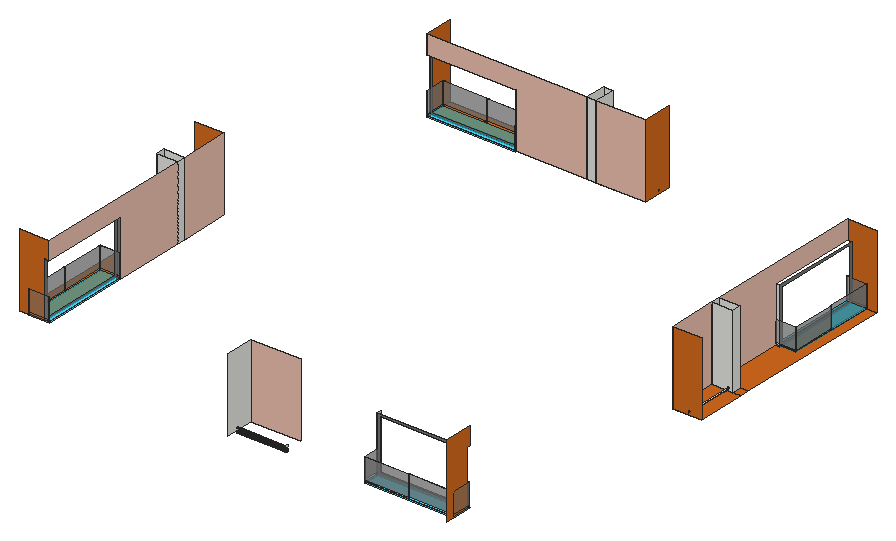
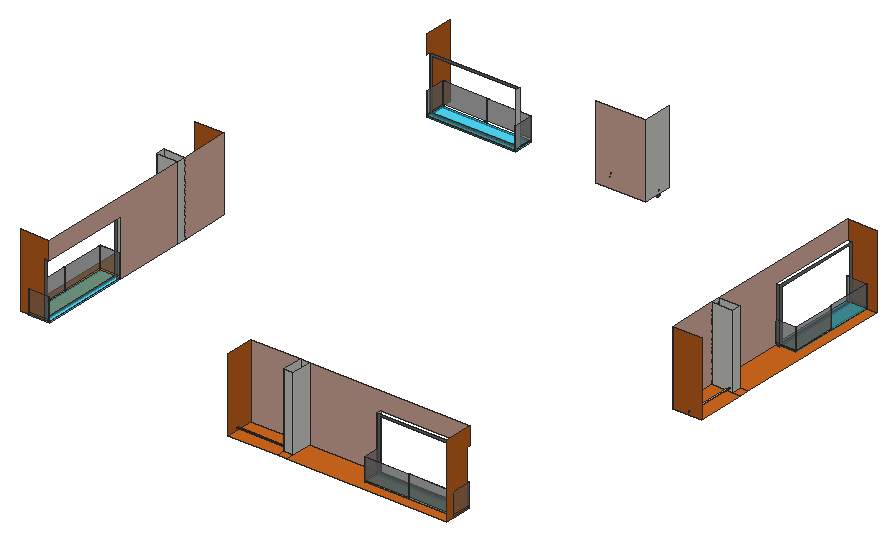
# SketchUp Ruby script. Lengths in inches.
U = 1.inch
M = Sketchup.active_model
def pt(a) = Geom::Point3d.new(a.map { |v| v * U })
def face(e, loops, mat)
  f = e.add_face(loops[0].map { |a| pt(a) })
  loops[1..].each { |l| e.add_face(l.map { |a| pt(a) }).erase! }
  f.material = f.back_material = mat if mat
  f
end
# faces: each face lists its corners as indices into pts; further lists are holes
def faces(e, pts, list, mat = nil) = list.each { |f| face(e, (f[0].is_a?(Array) ? f : [f]).map { |l| l.map { |i| pts[i] } }, mat) }
# xy, xz, yz: faces in a plane at the given z, y or x. An outline is a flat list of corners, or four numbers for a rectangle; further outlines are holes
def ring(l) = l.size == 4 ? [[l[0], l[1]], [l[2], l[1]], [l[2], l[3]], [l[0], l[3]]] : l.each_slice(2).to_a
def flat(e, list, mat, &to3) = list.each { |f| face(e, (f[0].is_a?(Array) ? f : [f]).map { |l| ring(l).map { |u, v| to3.(u, v) } }, mat) }
def xy(e, z, list, mat = nil) = flat(e, list, mat) { |x, y| [x, y, z] }
def xz(e, y, list, mat = nil) = flat(e, list, mat) { |x, z| [x, y, z] }
def yz(e, x, list, mat = nil) = flat(e, list, mat) { |y, z| [x, y, z] }
def lines(e, pts, list) = list.each { |a, b| e.add_line(pt(pts[a]), pt(pts[b])) }
# prism: a flat outline (further loops are holes) pulled along v
def prism(e, loops, v, mat = nil)
  f = face(e, loops, mat); d = Geom::Vector3d.new(v.map { |x| x * U })
  f.pushpull(f.normal.samedirection?(d) ? d.length : -d.length)
end
def box(e, o, s, mat = nil) = prism(e, [[o, [o[0] + s[0], o[1], o[2]], [o[0] + s[0], o[1] + s[1], o[2]], [o[0], o[1] + s[1], o[2]]]], [0, 0, s[2]], mat)
def at(x, y, z, deg = 0) = Geom::Transformation.translation(pt([x, y, z])) * Geom::Transformation.rotation(ORIGIN, Z_AXIS, deg.degrees)
def axes(o, x, y, z) = Geom::Transformation.new([*x, 0, *y, 0, *z, 0, *pt(o).to_a, 1])
def part(name) = M.definitions.add(name)
# library, detail: a bought-in or finely detailed component or shape, given as its bounding box
def library(name, o, s) = part(name).tap { |d| box(d.entities, o, s) }
def detail(e, o, s) = box(e.add_group.entities, o, s)
def put(e, d, t, mat = nil) = e.add_instance(d, t).tap { |i| i.material = mat if mat }
def group(e, t, mat = nil) = e.add_group.tap { |g| g.transformation = t; g.material = mat if mat }.entities
root = M.entities
M.materials.add("[0041_Chocolate]").color = [210, 105, 30]
M.materials.add("[0042_Sienna]").color = [160, 82, 45]
M.materials.add("[0119_RosyBrown]").color = [234, 190, 174]
M.materials.add("[Metal Seamed]").color = [118, 119, 115]
M.materials.add("[Translucent Glass Tinted]").color = [8, 201, 241]
M.materials["[Translucent Glass Tinted]"].alpha = 0.48
M.materials.add("[Translucent_Glass_Gray]").color = [128, 128, 128]
M.materials["[Translucent_Glass_Gray]"].alpha = 0.5
c1 = part("Altan")
box(c1.entities,[0,0,0],[118.11,59.06,3.9375])
c2 = part("Staal sojle alta")
box(c2.entities,[0,0,0],[0.87,0.87,43.31])
c3 = part("gler")
box(c3.entities,[0,-0.71,0],[0.37,57.8,41.34],"[Translucent_Glass_Gray]")
xy(root,1573.11,[[72,636.29,132,662.8],[1488,886.83,1548,913.33],[671.48,1452.8125,697.99,1512.8125]])
xy(root,1573.11,[[48,169.92,120,169.92,120,429.61,132,429.61,132,636.29,48,636.29],[48,636.29,72,662.8],[48,662.8,132,806.17],[1488,743.45,1572,886.83],[1548,886.83,1572,913.33],
  [1488,913.33,1572,913.33,1572,1379.7,1500,1379.7,1500,1120.01,1488,1120.01],[464.8,1452.8125,671.48,1452.8125,671.48,1536.8125,205.11,1536.8125,205.11,1464.8125,464.8,1464.8125],[697.99,1452.8125,841.36,1536.8125],[671.48,1512.8125,697.99,1536.8125]],"[0041_Chocolate]")
xy(root,1573.11,[[1155.2,84.8125,1414.89,96.8125]],"[0042_Sienna]")
xz(root,84.8125,[[[1155.2,1573.11,1414.89,1733.61],[1161.2,1579.11,1408.89,1727.61]]],"[Metal Seamed]")
xz(root,96.8125,[[778.64,1573.11,922.01,1786.89]],"[0119_RosyBrown]")
xz(root,169.92,[[48,1573.11,48,1786.89,132,1786.89,132,1733.61,120,1733.61,120,1573.11]],"[0041_Chocolate]")
xz(root,429.61,[[120,1573.11,132,1733.61]],"[Metal Seamed]")
xz(root,636.29,[[72,1573.11,132,1786.89]])
xz(root,662.8,[[[72,1573.11,132,1786.89],[83.53,1578.02,84.48,1578.14,85.37,1578.51,86.13,1579.1,86.72,1579.86,87.09,1580.75,87.21,1581.7,87.09,1582.66,86.72,1583.55,86.13,1584.3125,85.37,1584.9,84.48,1585.27,83.53,1585.39,82.57,1585.27,81.68,1584.9,80.92,1584.3125,80.33,1583.55,79.97,1582.66,79.84,1581.7,79.97,1580.75,80.33,1579.86,80.92,1579.1,81.68,1578.51,82.57,1578.14]],[83.53,1578.02,84.48,1578.14,85.37,1578.51,86.13,1579.1,86.72,1579.86,87.09,1580.75,87.21,1581.7,87.09,1582.66,86.72,1583.55,86.13,1584.3125,85.37,1584.9,84.48,1585.27,83.53,1585.39,82.57,1585.27,81.68,1584.9,80.92,1584.3125,80.33,1583.55,79.97,1582.66,79.84,1581.7,79.97,1580.75,80.33,1579.86,80.92,1579.1,81.68,1578.51,82.57,1578.14]])
xz(root,743.45,[[[1488,1573.11,1572,1786.89],[1536.47,1578.02,1537.43,1578.14,1538.32,1578.51,1539.08,1579.1,1539.67,1579.86,1540.03,1580.75,1540.16,1581.7,1540.03,1582.66,1539.67,1583.55,1539.08,1584.3125,1538.32,1584.9,1537.43,1585.27,1536.47,1585.39,1535.52,1585.27,1534.63,1584.9,1533.87,1584.3125,1533.28,1583.55,1532.91,1582.66,1532.79,1581.7,1532.91,1580.75,1533.28,1579.86,1533.87,1579.1,1534.63,1578.51,1535.52,1578.14]]],"[0041_Chocolate]")
xz(root,806.17,[[[48,1573.11,132,1786.89],[83.53,1578.02,82.57,1578.14,81.68,1578.51,80.92,1579.1,80.33,1579.86,79.97,1580.75,79.84,1581.7,79.97,1582.66,80.33,1583.55,80.92,1584.3125,81.68,1584.9,82.57,1585.27,83.53,1585.39,84.48,1585.27,85.37,1584.9,86.13,1584.3125,86.72,1583.55,87.09,1582.66,87.21,1581.7,87.09,1580.75,86.72,1579.86,86.13,1579.1,85.37,1578.51,84.48,1578.14]]],"[0041_Chocolate]")
xz(root,886.83,[[[1488,1573.11,1548,1786.89],[1536.47,1578.02,1535.52,1578.14,1534.63,1578.51,1533.87,1579.1,1533.28,1579.86,1532.91,1580.75,1532.79,1581.7,1532.91,1582.66,1533.28,1583.55,1533.87,1584.3125,1534.63,1584.9,1535.52,1585.27,1536.47,1585.39,1537.43,1585.27,1538.32,1584.9,1539.08,1584.3125,1539.67,1583.55,1540.03,1582.66,1540.16,1581.7,1540.03,1580.75,1539.67,1579.86,1539.08,1579.1,1538.32,1578.51,1537.43,1578.14]],[1536.47,1578.02,1535.52,1578.14,1534.63,1578.51,1533.87,1579.1,1533.28,1579.86,1532.91,1580.75,1532.79,1581.7,1532.91,1582.66,1533.28,1583.55,1533.87,1584.3125,1534.63,1584.9,1535.52,1585.27,1536.47,1585.39,1537.43,1585.27,1538.32,1584.9,1539.08,1584.3125,1539.67,1583.55,1540.03,1582.66,1540.16,1581.7,1540.03,1580.75,1539.67,1579.86,1539.08,1579.1,1538.32,1578.51,1537.43,1578.14]])
xz(root,913.33,[[1488,1573.11,1548,1786.89]])
xz(root,1120.01,[[1488,1573.11,1500,1733.61]])
xz(root,1379.7,[[1500,1573.11,1572,1573.11,1572,1786.89,1488,1786.89,1488,1733.61,1500,1733.61]],"[0041_Chocolate]")
xz(root,1452.8125,[[671.48,1573.11,697.99,1786.89]])
xz(root,1452.8125,[[464.8,1573.11,464.8,1733.61,205.11,1733.61,205.11,1786.89,671.48,1786.89,671.48,1573.11],[697.99,1573.11,841.36,1786.89]],"[0119_RosyBrown]")
xz(root,1464.8125,[[[205.11,1573.11,464.8,1733.61],[211.11,1579.11,458.8,1727.61]]],"[Metal Seamed]")
xz(root,1512.8125,[[671.48,1573.11,697.99,1786.89]])
yz(root,72,[[636.29,1573.11,662.8,1786.89]])
yz(root,120,[[[169.92,1573.11,429.61,1733.61],[175.92,1579.11,423.61,1727.61]]],"[Metal Seamed]")
yz(root,132,[[636.29,1573.11,662.8,1786.89]])
yz(root,132,[[429.61,1573.11,429.61,1733.61,169.92,1733.61,169.92,1786.89,636.29,1786.89,636.29,1573.11],[662.8,1573.11,806.17,1786.89]],"[0119_RosyBrown]")
yz(root,205.11,[[1464.8125,1573.11,1536.8125,1573.11,1536.8125,1786.89,1452.8125,1786.89,1452.8125,1733.61,1464.8125,1733.61]],"[0041_Chocolate]")
yz(root,464.8,[[1452.8125,1573.11,1464.8125,1733.61]])
yz(root,671.48,[[1452.8125,1573.11,1512.8125,1786.89]])
yz(root,697.99,[[[1452.8125,1573.11,1512.8125,1786.89],[1501.28,1578.02,1500.33,1578.14,1499.44,1578.51,1498.68,1579.1,1498.09,1579.86,1497.72,1580.75,1497.6,1581.7,1497.72,1582.66,1498.09,1583.55,1498.68,1584.3125,1499.44,1584.9,1500.33,1585.27,1501.28,1585.39,1502.24,1585.27,1503.13,1584.9,1503.89,1584.3125,1504.48,1583.55,1504.85,1582.66,1504.97,1581.7,1504.85,1580.75,1504.48,1579.86,1503.89,1579.1,1503.13,1578.51,1502.24,1578.14]],[1501.28,1578.02,1500.33,1578.14,1499.44,1578.51,1498.68,1579.1,1498.09,1579.86,1497.72,1580.75,1497.6,1581.7,1497.72,1582.66,1498.09,1583.55,1498.68,1584.3125,1499.44,1584.9,1500.33,1585.27,1501.28,1585.39,1502.24,1585.27,1503.13,1584.9,1503.89,1584.3125,1504.48,1583.55,1504.85,1582.66,1504.97,1581.7,1504.85,1580.75,1504.48,1579.86,1503.89,1579.1,1503.13,1578.51,1502.24,1578.14]])
yz(root,778.64,[[[12.8125,1573.11,47.01,1573.11,47.38,1573.27,48.34,1573.39,49.29,1573.27,49.67,1573.11,96.8125,1573.11,96.8125,1786.89,12.8125,1786.89],[48.34,1578.02,47.38,1578.14,46.5,1578.51,45.73,1579.1,45.15,1579.86,44.78,1580.75,44.65,1581.7,44.78,1582.66,45.15,1583.55,45.73,1584.3125,46.5,1584.9,47.38,1585.27,48.34,1585.39,49.29,1585.27,50.18,1584.9,50.95,1584.3125,51.53,1583.55,51.9,1582.66,52.03,1581.7,51.9,1580.75,51.53,1579.86,50.95,1579.1,50.18,1578.51,49.29,1578.14]],[47.01,1573.11,49.67,1573.11,49.29,1573.27,48.34,1573.39,47.38,1573.27]])
yz(root,778.64,[[48.34,1566.02,49.29,1566.14,50.18,1566.51,50.95,1567.1,51.53,1567.86,51.9,1568.75,52.03,1569.7,51.9,1570.66,51.53,1571.55,50.95,1572.3125,50.18,1572.9,49.67,1573.11,47.01,1573.11,46.5,1572.9,45.73,1572.3125,45.15,1571.55,44.78,1570.66,44.65,1569.7,44.78,1568.75,45.15,1567.86,45.73,1567.1,46.5,1566.51,47.38,1566.14]],"[0042_Sienna]")
yz(root,841.36,[[[1452.8125,1573.11,1536.8125,1786.89],[1501.28,1578.02,1502.24,1578.14,1503.13,1578.51,1503.89,1579.1,1504.48,1579.86,1504.85,1580.75,1504.97,1581.7,1504.85,1582.66,1504.48,1583.55,1503.89,1584.3125,1503.13,1584.9,1502.24,1585.27,1501.28,1585.39,1500.33,1585.27,1499.44,1584.9,1498.68,1584.3125,1498.09,1583.55,1497.72,1582.66,1497.6,1581.7,1497.72,1580.75,1498.09,1579.86,1498.68,1579.1,1499.44,1578.51,1500.33,1578.14]]],"[0041_Chocolate]")
yz(root,922.01,[[48.34,1578.02,49.29,1578.14,50.18,1578.51,50.95,1579.1,51.53,1579.86,51.9,1580.75,52.03,1581.7,51.9,1582.66,51.53,1583.55,50.95,1584.3125,50.18,1584.9,49.29,1585.27,48.34,1585.39,47.38,1585.27,46.5,1584.9,45.73,1584.3125,45.15,1583.55,44.78,1582.66,44.65,1581.7,44.78,1580.75,45.15,1579.86,45.73,1579.1,46.5,1578.51,47.38,1578.14]])
yz(root,1155.2,[[84.8125,1573.11,96.8125,1733.61]])
yz(root,1414.89,[[12.8125,1573.11,12.8125,1786.89,96.8125,1786.89,96.8125,1733.61,84.8125,1733.61,84.8125,1573.11]],"[0041_Chocolate]")
yz(root,1488,[[886.83,1573.11,913.33,1786.89]])
yz(root,1488,[[743.45,1573.11,886.83,1786.89],[913.33,1573.11,1120.01,1573.11,1120.01,1733.61,1379.7,1733.61,1379.7,1786.89,913.33,1786.89]],"[0119_RosyBrown]")
yz(root,1500,[[[1120.01,1573.11,1379.7,1733.61],[1126.01,1579.11,1373.7,1727.61]]],"[Metal Seamed]")
yz(root,1548,[[886.83,1573.11,913.33,1786.89]])
p = [[922.01,48.34,1566.02],[922.01,47.38,1566.14],[778.64,47.38,1566.14],[778.64,48.34,1566.02],[922.01,49.29,1566.14],[778.64,49.29,1566.14],
  [922.01,46.5,1566.51],[778.64,46.5,1566.51],[922.01,50.18,1566.51],[778.64,50.18,1566.51],[922.01,45.73,1567.1],[778.64,45.73,1567.1],
  [922.01,50.95,1567.1],[778.64,50.95,1567.1],[922.01,45.15,1567.86],[778.64,45.15,1567.86],[922.01,51.53,1567.86],[778.64,51.53,1567.86],
  [922.01,44.78,1568.75],[778.64,44.78,1568.75],[922.01,51.9,1568.75],[778.64,51.9,1568.75],[922.01,44.65,1569.7],[778.64,44.65,1569.7],
  [922.01,52.03,1569.7],[778.64,52.03,1569.7],[922.01,44.78,1570.66],[778.64,44.78,1570.66],[922.01,51.9,1570.66],[778.64,51.9,1570.66],
  [922.01,45.15,1571.55],[778.64,45.15,1571.55],[922.01,51.53,1571.55],[778.64,51.53,1571.55],[922.01,45.73,1572.3125],[778.64,45.73,1572.3125],
  [922.01,50.95,1572.3125],[778.64,50.95,1572.3125],[922.01,46.5,1572.9],[778.64,46.5,1572.9],[922.01,50.18,1572.9],[778.64,50.18,1572.9],
  [922.01,47.38,1573.27],[778.64,47.38,1573.27],[778.64,47.01,1573.11],[922.01,49.29,1573.27],[778.64,49.67,1573.11],[778.64,49.29,1573.27],
  [922.01,48.34,1573.39],[778.64,48.34,1573.39],[922.01,48.34,1578.02],[922.01,47.38,1578.14],[778.64,47.38,1578.14],[778.64,48.34,1578.02],
  [922.01,49.29,1578.14],[778.64,49.29,1578.14],[83.53,662.8,1578.02],[82.57,662.8,1578.14],[82.57,806.17,1578.14],[83.53,806.17,1578.02],
  [84.48,662.8,1578.14],[84.48,806.17,1578.14],[1535.52,886.83,1578.14],[1536.47,886.83,1578.02],[1536.47,743.45,1578.02],[1535.52,743.45,1578.14],
  [1537.43,886.83,1578.14],[1537.43,743.45,1578.14],[697.99,1500.33,1578.14],[697.99,1501.28,1578.02],[841.36,1501.28,1578.02],[841.36,1500.33,1578.14],
  [697.99,1502.24,1578.14],[841.36,1502.24,1578.14],[922.01,46.5,1578.51],[778.64,46.5,1578.51],[922.01,50.18,1578.51],[778.64,50.18,1578.51],
  [81.68,662.8,1578.51],[81.68,806.17,1578.51],[85.37,662.8,1578.51],[85.37,806.17,1578.51],[1534.63,886.83,1578.51],[1534.63,743.45,1578.51],
  [1538.32,886.83,1578.51],[1538.32,743.45,1578.51],[697.99,1499.44,1578.51],[841.36,1499.44,1578.51],[697.99,1503.13,1578.51],[841.36,1503.13,1578.51],
  [922.01,45.73,1579.1],[778.64,45.73,1579.1],[922.01,50.95,1579.1],[778.64,50.95,1579.1],[80.92,662.8,1579.1],[80.92,806.17,1579.1],
  [86.13,662.8,1579.1],[86.13,806.17,1579.1],[1533.87,886.83,1579.1],[1533.87,743.45,1579.1],[1539.08,886.83,1579.1],[1539.08,743.45,1579.1],
  [697.99,1498.68,1579.1],[841.36,1498.68,1579.1],[697.99,1503.89,1579.1],[841.36,1503.89,1579.1]]
faces(root,p,[[0,1,2,3],[4,0,3,5],[1,6,7,2],[8,4,5,9],[6,10,11,7],[12,8,9,13],[10,14,15,11],[16,12,13,17],
  [14,18,19,15],[20,16,17,21],[18,22,23,19],[24,20,21,25],[22,26,27,23],[28,24,25,29],[26,30,31,27],[32,28,29,33],
  [30,34,35,31],[36,32,33,37],[34,38,39,35],[40,36,37,41],[38,42,43,44,39],[45,40,41,46,47],[42,48,49,43],[48,45,47,49],
  [50,51,52,53],[54,50,53,55],[56,57,58,59],[60,56,59,61],[62,63,64,65],[63,66,67,64],[68,69,70,71],[69,72,73,70],
  [51,74,75,52],[76,54,55,77],[57,78,79,58],[80,60,61,81],[82,62,65,83],[66,84,85,67],[86,68,71,87],[72,88,89,73],
  [74,90,91,75],[92,76,77,93],[78,94,95,79],[96,80,81,97],[98,82,83,99],[84,100,101,85],[102,86,87,103],[88,104,105,89]])
put(root,c1,axes([205.11,1451.94,1569.17],[2.19843,0,0],[0,1,0],[0,0,1.5]),"[Translucent Glass Tinted]")
put(root,c1,axes([1414.89,97.68,1569.17],[-2.19843,0,0],[0,-1,0],[0,0,1.5]),"[Translucent Glass Tinted]")
put(root,c1,axes([1487.13,1379.7,1569.17],[0,-2.19843,0],[1,0,0],[0,0,1.5]),"[Translucent Glass Tinted]")
put(root,c1,axes([132.87,169.92,1569.17],[0,2.19843,0],[-1,0,0],[0,0,1.5]),"[Translucent Glass Tinted]")
put(root,c2,axes([462.85,1510.125,1575.08],[2.19843,0,0],[0,1,0],[0,0,1.5]),"[Translucent Glass Tinted]")
put(root,c2,axes([1286.12,39.5,1575.08],[-2.19843,0,0],[0,-1,0],[0,0,1.5]),"[Translucent Glass Tinted]")
put(root,c2,axes([205.11,1451.94,1575.08],[2.19843,0,0],[0,1,0],[0,0,1.5]),"[Translucent Glass Tinted]")
put(root,c2,axes([1414.89,97.68,1575.08],[-2.19843,0,0],[0,-1,0],[0,0,1.5]),"[Translucent Glass Tinted]")
put(root,c2,axes([462.85,1451.94,1575.08],[2.19843,0,0],[0,1,0],[0,0,1.5]),"[Translucent Glass Tinted]")
put(root,c2,axes([205.11,1510.125,1575.08],[2.19843,0,0],[0,1,0],[0,0,1.5]),"[Translucent Glass Tinted]")
put(root,c2,axes([74.69,427.66,1575.08],[0,2.19843,0],[-1,0,0],[0,0,1.5]),"[Translucent Glass Tinted]")
put(root,c2,axes([1157.15,97.68,1575.08],[-2.19843,0,0],[0,-1,0],[0,0,1.5]),"[Translucent Glass Tinted]")
put(root,c2,axes([1414.89,39.5,1575.08],[-2.19843,0,0],[0,-1,0],[0,0,1.5]),"[Translucent Glass Tinted]")
put(root,c2,axes([132.87,427.66,1575.08],[0,2.19843,0],[-1,0,0],[0,0,1.5]),"[Translucent Glass Tinted]")
put(root,c2,axes([132.87,169.92,1575.08],[0,2.19843,0],[-1,0,0],[0,0,1.5]),"[Translucent Glass Tinted]")
put(root,c2,axes([333.88,1510.125,1575.08],[2.19843,0,0],[0,1,0],[0,0,1.5]),"[Translucent Glass Tinted]")
put(root,c2,axes([74.69,169.92,1575.08],[0,2.19843,0],[-1,0,0],[0,0,1.5]),"[Translucent Glass Tinted]")
put(root,c2,axes([1487.13,1121.96,1575.08],[0,-2.19843,0],[1,0,0],[0,0,1.5]),"[Translucent Glass Tinted]")
put(root,c2,axes([1545.31,1250.93,1575.08],[0,-2.19843,0],[1,0,0],[0,0,1.5]),"[Translucent Glass Tinted]")
put(root,c2,axes([1545.31,1121.96,1575.08],[0,-2.19843,0],[1,0,0],[0,0,1.5]),"[Translucent Glass Tinted]")
put(root,c2,axes([1545.31,1379.7,1575.08],[0,-2.19843,0],[1,0,0],[0,0,1.5]),"[Translucent Glass Tinted]")
put(root,c2,axes([1157.15,39.5,1575.08],[-2.19843,0,0],[0,-1,0],[0,0,1.5]),"[Translucent Glass Tinted]")
put(root,c2,axes([74.69,298.69,1575.08],[0,2.19843,0],[-1,0,0],[0,0,1.5]),"[Translucent Glass Tinted]")
put(root,c2,axes([1487.13,1379.7,1575.08],[0,-2.19843,0],[1,0,0],[0,0,1.5]),"[Translucent Glass Tinted]")
put(root,c3,axes([337.35,1511,1578.03],[0,-1,0],[2.19843,0,0],[0,0,1.5]),"[Translucent Glass Tinted]")
put(root,c3,axes([1411.62,38.625,1578.03],[0,1,0],[-2.19843,0,0],[0,0,1.5]),"[Translucent Glass Tinted]")
put(root,c3,axes([1282.65,38.625,1578.03],[0,1,0],[-2.19843,0,0],[0,0,1.5]),"[Translucent Glass Tinted]")
put(root,c3,axes([131.77,428.84,1578.03],[0,2.19843,0],[-1,0,0],[0,0,1.5]),"[Translucent Glass Tinted]")
put(root,c3,axes([1414.89,96.58,1578.03],[-2.19843,0,0],[0,-1,0],[0,0,1.5]),"[Translucent Glass Tinted]")
put(root,c3,axes([1155.97,96.58,1578.03],[-2.19843,0,0],[0,-1,0],[0,0,1.5]),"[Translucent Glass Tinted]")
put(root,c3,axes([205.11,1453.04,1578.03],[2.19843,0,0],[0,1,0],[0,0,1.5]),"[Translucent Glass Tinted]")
put(root,c3,axes([131.77,169.92,1578.03],[0,2.19843,0],[-1,0,0],[0,0,1.5]),"[Translucent Glass Tinted]")
put(root,c3,axes([464.03,1453.04,1578.03],[2.19843,0,0],[0,1,0],[0,0,1.5]),"[Translucent Glass Tinted]")
put(root,c3,axes([73.81,173.19,1578.03],[1,0,0],[0,2.19843,0],[0,0,1.5]),"[Translucent Glass Tinted]")
put(root,c3,axes([208.38,1511,1578.03],[0,-1,0],[2.19843,0,0],[0,0,1.5]),"[Translucent Glass Tinted]")
put(root,c3,axes([73.81,302.16,1578.03],[1,0,0],[0,2.19843,0],[0,0,1.5]),"[Translucent Glass Tinted]")
put(root,c3,axes([1546.19,1247.46,1578.03],[-1,0,0],[0,-2.19843,0],[0,0,1.5]),"[Translucent Glass Tinted]")
put(root,c3,axes([1488.23,1379.7,1578.03],[0,-2.19843,0],[1,0,0],[0,0,1.5]),"[Translucent Glass Tinted]")
put(root,c3,axes([1546.19,1376.43,1578.03],[-1,0,0],[0,-2.19843,0],[0,0,1.5]),"[Translucent Glass Tinted]")
put(root,c3,axes([1488.23,1120.78,1578.03],[0,-2.19843,0],[1,0,0],[0,0,1.5]),"[Translucent Glass Tinted]")
